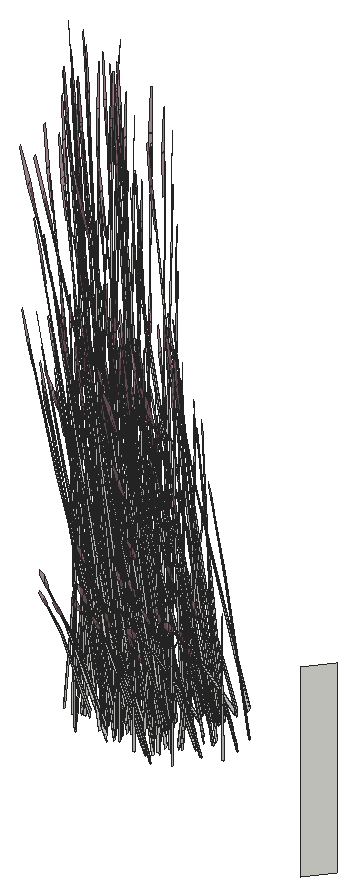
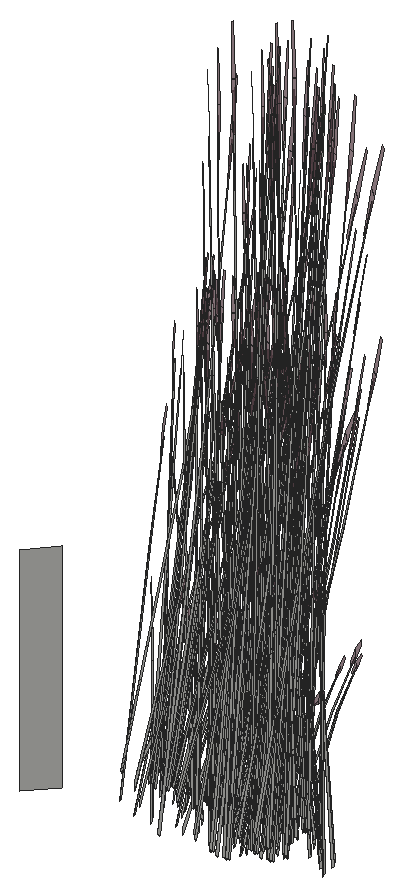
# SketchUp Ruby script. Lengths in inches.
U = 1.inch
M = Sketchup.active_model
def pt(a) = Geom::Point3d.new(a.map { |v| v * U })
def face(e, loops, mat)
  f = e.add_face(loops[0].map { |a| pt(a) })
  loops[1..].each { |l| e.add_face(l.map { |a| pt(a) }).erase! }
  f.material = f.back_material = mat if mat
  f
end
# faces: each face lists its corners as indices into pts; further lists are holes
def faces(e, pts, list, mat = nil) = list.each { |f| face(e, (f[0].is_a?(Array) ? f : [f]).map { |l| l.map { |i| pts[i] } }, mat) }
# xy, xz, yz: faces in a plane at the given z, y or x. An outline is a flat list of corners, or four numbers for a rectangle; further outlines are holes
def ring(l) = l.size == 4 ? [[l[0], l[1]], [l[2], l[1]], [l[2], l[3]], [l[0], l[3]]] : l.each_slice(2).to_a
def flat(e, list, mat, &to3) = list.each { |f| face(e, (f[0].is_a?(Array) ? f : [f]).map { |l| ring(l).map { |u, v| to3.(u, v) } }, mat) }
def xy(e, z, list, mat = nil) = flat(e, list, mat) { |x, y| [x, y, z] }
def xz(e, y, list, mat = nil) = flat(e, list, mat) { |x, z| [x, y, z] }
def yz(e, x, list, mat = nil) = flat(e, list, mat) { |y, z| [x, y, z] }
def lines(e, pts, list) = list.each { |a, b| e.add_line(pt(pts[a]), pt(pts[b])) }
# prism: a flat outline (further loops are holes) pulled along v
def prism(e, loops, v, mat = nil)
  f = face(e, loops, mat); d = Geom::Vector3d.new(v.map { |x| x * U })
  f.pushpull(f.normal.samedirection?(d) ? d.length : -d.length)
end
def box(e, o, s, mat = nil) = prism(e, [[o, [o[0] + s[0], o[1], o[2]], [o[0] + s[0], o[1] + s[1], o[2]], [o[0], o[1] + s[1], o[2]]]], [0, 0, s[2]], mat)
def at(x, y, z, deg = 0) = Geom::Transformation.translation(pt([x, y, z])) * Geom::Transformation.rotation(ORIGIN, Z_AXIS, deg.degrees)
def axes(o, x, y, z) = Geom::Transformation.new([*x, 0, *y, 0, *z, 0, *pt(o).to_a, 1])
def part(name) = M.definitions.add(name)
# library, detail: a bought-in or finely detailed component or shape, given as its bounding box
def library(name, o, s) = part(name).tap { |d| box(d.entities, o, s) }
def detail(e, o, s) = box(e.add_group.entities, o, s)
def put(e, d, t, mat = nil) = e.add_instance(d, t).tap { |i| i.material = mat if mat }
def group(e, t, mat = nil) = e.add_group.tap { |g| g.transformation = t; g.material = mat if mat }.entities
root = M.entities
M.materials.add("LightPink_Translucent").color = [144, 107, 117]
M.materials["LightPink_Translucent"].alpha = 0.75
c1 = part("blade")
p = [[2.15,0.21,22],[0,0.17,0],[0.09,0.45,0],[2.18,0.31,22],[2.29,0.31,22],[0.38,0.45,0],
  [2.48,0.24,33],[2.49,0.24,33],[2.48,0.22,33]]
faces(c1.entities,p,[[0,1,2,3],[4,5,2,3],[6,3,4,7],[8,0,3,6]])
c2 = part("seeds")
p = [[0.3,-0.1,1.38],[-0.01,-0.03,1.59],[-0.01,-0.03,0.03],[0.14,-0.07,-0.07],[0.29,-0.03,3],[0.15,0.01,3.11]]
faces(c2.entities,p,[[0,1,2,3],[1,0,4,5]],"LightPink_Translucent")
c3 = part("blade with seeds")
put(c3.entities,c1,at(0,0,0))
put(c3.entities,c2,axes([2.4,0.25,30.99],[1.5799,-0.05474,1.17369],[-0.12525,1.92788,0.29478],[-0.07173,-0.02425,1.56792]))
p = [[371.24,649.12,618],[369.42,647.05,618],[369.42,647.05,636],[371.24,649.12,636]]
faces(root,p,[[0,1,2,3]])
put(root,c3,axes([347.8,648.96,622.99],[0.18411,0.16231,1.1486],[-0.26813,0.09757,0.84392],[-0.05737,-0.12474,0.25299]))
put(root,c3,axes([349.17,649.44,624.96],[0.26007,-0.1585,0.0643],[0.12729,0.28902,0.50621],[-0.02512,-0.1274,0.77189]))
put(root,c3,axes([349.38,649.62,624.78],[0.39316,-0.11987,0.53763],[0.06823,0.47021,0.4433],[-0.09247,-0.13858,1.11249]))
put(root,c3,axes([352.93,649.92,620.63],[-0.0592,0.0168,1.76342],[-0.32738,-0.18913,-0.26939],[0.00549,-0.15776,0.30037]))
put(root,c3,axes([350.27,649.71,624.42],[0.34777,0.12192,0.48003],[-0.11892,0.40083,0.3958],[-0.0209,-0.15763,0.9933]))
put(root,c3,axes([350.37,649.85,624.73],[-0.34538,0.21713,-0.1216],[-0.16972,-0.38536,-0.67495],[-0.04557,-0.16239,1.02557]))
put(root,c3,axes([351.09,650.34,624.73],[-0.3879,-0.02311,-0.1216],[0.0106,-0.43749,-0.67495],[0.02694,-0.1685,1.02557]))
put(root,c3,axes([351.0625,650.06,624.22],[0.23881,-0.24554,-0.35414],[0.22606,0.28036,0.4572],[0.0344,-0.14245,0.87481]))
put(root,c3,axes([349,649.19,622.46],[0.18411,0.16231,1.1486],[-0.26813,0.09757,0.84392],[-0.05737,-0.12474,0.25299]))
put(root,c3,axes([350.36,649.68,624.42],[0.26007,-0.1585,0.0643],[0.12729,0.28902,0.50621],[-0.02512,-0.1274,0.77189]))
put(root,c3,axes([353.92,651.13,624.12],[0.00918,-0.43138,-0.71045],[0.38672,0.02897,0.08574],[0.04081,-0.18275,1.00501]))
put(root,c3,axes([349.44,650.05,624.67],[-0.30095,-0.22541,-0.71045],[0.21388,-0.395,0.08574],[-0.10904,-0.13459,1.00501]))
put(root,c3,axes([349.34,649.76,624.22],[-0.05451,-0.37564,-0.35414],[0.31161,-0.09919,0.4572],[-0.0837,-0.10765,0.87481]))
put(root,c3,axes([354.46,650.46,623.85],[-0.00341,-0.09282,1.74944],[-0.28775,-0.26825,-0.27667],[0.04449,-0.16261,0.14031]))
put(root,c3,axes([353.25,650.4375,623.66],[0.1064,-0.35863,-0.35414],[0.31043,0.1046,0.4572],[-0.02846,-0.14439,0.87481]))
put(root,c3,axes([353.48,650.91,623.01],[-0.06572,0.16029,1.71376],[-0.27569,-0.33172,0.13857],[0.12437,-0.20675,0.73262]))
put(root,c3,axes([354.38,650.125,623.85],[-0.03584,0.03562,1.77383],[-0.35118,-0.12018,-0.16761],[-0.01271,-0.15545,0.31391]))
put(root,c3,axes([346.05,649.49,621.22],[-0.05283,-0.03674,1.76342],[-0.13569,-0.41045,-0.26939],[0.09154,-0.11138,0.30037]))
put(root,c3,axes([348.28,649.48,624.96],[0.16041,-0.29625,0.0643],[0.22843,0.17248,0.50621],[-0.07385,-0.09498,0.77189]))
put(root,c3,axes([348.23,651.13,622.32],[-0.14494,-0.47823,-0.69835],[0.41752,-0.17223,-0.18329],[-0.01602,-0.16194,1.54149]))
put(root,c3,axes([353.09,650.68,623.82],[-0.34695,-0.11691,-0.51099],[0.11892,-0.40083,-0.3958],[-0.03181,-0.16138,0.97773]))
put(root,c3,axes([350.17,649.67,621.72],[-0.05283,-0.03674,1.76342],[-0.13569,-0.41045,-0.26939],[0.09154,-0.11138,0.30037]))
put(root,c3,axes([353.31,649.68,621.9],[0.04528,0.27194,1.1486],[-0.25117,-0.15062,0.84392],[0.02703,-0.13924,0.25299]))
put(root,c3,axes([345.75,649.74,624.46],[0.25132,0.3182,0.48003],[-0.2669,0.27442,0.3958],[0.04636,-0.14929,0.9933]))
put(root,c3,axes([353.84,650.99,623.82],[-0.25266,-0.31335,-0.51099],[0.2669,-0.27442,-0.3958],[0.03844,-0.15921,0.97773]))
put(root,c3,axes([349.47,649.72,624.42],[0.16041,-0.29625,0.0643],[0.22843,0.17248,0.50621],[-0.07385,-0.09498,0.77189]))
put(root,c3,axes([348.85,649.68,621.18],[-0.03419,0.06144,1.76342],[-0.3455,0.13246,-0.26939],[-0.08346,-0.12049,0.30037]))
put(root,c3,axes([349.07,649.77,625.28],[-0.1064,0.35863,0.35414],[-0.31043,-0.1046,-0.4572],[-0.02846,-0.14439,0.87481]))
put(root,c3,axes([352.47,649.44,623.85],[-0.00658,0.0559,1.77383],[-0.32474,0.20287,-0.16761],[-0.09556,-0.1037,0.31391]))
put(root,c3,axes([349.42,651.37,621.79],[-0.14494,-0.47823,-0.69835],[0.41752,-0.17223,-0.18329],[-0.01602,-0.16194,1.54149]))
put(root,c3,axes([349.87,649.92,624.96],[0.25132,0.3182,0.48003],[-0.2669,0.27442,0.3958],[0.04636,-0.14929,0.9933]))
put(root,c3,axes([351.36,649.91,621.18],[-0.05283,-0.03674,1.76342],[-0.13569,-0.41045,-0.26939],[0.09154,-0.11138,0.30037]))
put(root,c3,axes([346.05,650.65,624.71],[0.18436,-0.36797,-0.71045],[0.32306,0.26151,0.08574],[0.11008,-0.13332,1.00501]))
put(root,c3,axes([349.96,649.95,624.96],[0.29004,0.02173,0.0643],[-0.00795,0.32812,0.50621],[0.03035,-0.12569,0.77189]))
put(root,c3,axes([346.04,650.48,624.41],[-0.09067,-0.42583,-0.51099],[0.34336,-0.07449,-0.3958],[0.0984,-0.11438,0.97773]))
put(root,c3,axes([352.4,650.43,624.23],[0.39316,-0.11987,0.53763],[0.06823,0.47021,0.4433],[-0.09247,-0.13858,1.11249]))
put(root,c3,axes([350.27,650,624.74],[-0.1064,0.35863,0.35414],[-0.31043,-0.1046,-0.4572],[-0.02846,-0.14439,0.87481]))
put(root,c3,axes([349.74,650.17,625.28],[-0.23881,0.24554,0.35414],[-0.22606,-0.28036,-0.4572],[0.0344,-0.14245,0.87481]))
put(root,c3,axes([353.29,650.52,623.87],[0.34777,0.12192,0.48003],[-0.11892,0.40083,0.3958],[-0.0209,-0.15763,0.9933]))
put(root,c3,axes([350.16,650.83,625.21],[0.18436,-0.36797,-0.71045],[0.32306,0.26151,0.08574],[0.11008,-0.13332,1.00501]))
put(root,c3,axes([348.17,649.76,622.6],[-0.22066,-0.46731,0],[0.36918,-0.26061,-0.51607],[0.08408,-0.05936,1.63711]))
put(root,c3,axes([350.16,650.66,624.91],[-0.09067,-0.42583,-0.51099],[0.34336,-0.07449,-0.3958],[0.0984,-0.11438,0.97773]))
put(root,c3,axes([353.39,650.66,624.17],[-0.34538,0.21713,-0.1216],[-0.16972,-0.38536,-0.67495],[-0.04557,-0.16239,1.02557]))
put(root,c3,axes([349.3,650.07,624.37],[-0.34827,0.11086,-0.51099],[-0.06092,-0.41983,-0.3958],[-0.09354,-0.12031,0.97773]))
put(root,c3,axes([351.0625,650.15,624.42],[0.25132,0.3182,0.48003],[-0.2669,0.27442,0.3958],[0.04636,-0.14929,0.9933]))
put(root,c3,axes([354.11,651.15,624.17],[-0.3879,-0.02311,-0.1216],[0.0106,-0.43749,-0.67495],[0.02694,-0.1685,1.02557]))
put(root,c3,axes([346.2,650.78,624.76],[-0.32648,-0.25715,-0.1216],[0.18809,-0.3724,-0.67495],[0.09224,-0.12945,1.02557]))
put(root,c3,axes([349.55,649.69,625.12],[-0.23555,0.44708,-0.13619],[-0.34112,-0.25757,-0.75594],[-0.11858,-0.12631,1.14864]))
put(root,c3,axes([354.08,650.87,623.66],[0.23881,-0.24554,-0.35414],[0.22606,0.28036,0.4572],[0.0344,-0.14245,0.87481]))
put(root,c3,axes([352.01,650.01,621.9],[0.18411,0.16231,1.1486],[-0.26813,0.09757,0.84392],[-0.05737,-0.12474,0.25299]))
put(root,c3,axes([351.15,650.18,624.42],[0.29004,0.02173,0.0643],[-0.00795,0.32812,0.50621],[0.03035,-0.12569,0.77189]))
put(root,c3,axes([353.38,650.49,623.87],[0.26007,-0.1585,0.0643],[0.12729,0.28902,0.50621],[-0.02512,-0.1274,0.77189]))
put(root,c3,axes([348.66,649.2,622.35],[-0.2439,0.26754,-0.03893],[-0.22348,-0.29302,-0.17649],[-0.01573,-0.08303,0.58215]))
put(root,c3,axes([352.46,650.87,624.12],[-0.30095,-0.22541,-0.71045],[0.21388,-0.395,0.08574],[-0.10904,-0.13459,1.00501]))
put(root,c3,axes([352.35,650.57,623.66],[-0.05451,-0.37564,-0.35414],[0.31161,-0.09919,0.4572],[-0.0837,-0.10765,0.87481]))
put(root,c3,axes([350.9375,650.41,624.74],[-0.23881,0.24554,0.35414],[-0.22606,-0.28036,-0.4572],[0.0344,-0.14245,0.87481]))
put(root,c3,axes([350.32,650.96,625.26],[-0.32648,-0.25715,-0.1216],[0.18809,-0.3724,-0.67495],[0.09224,-0.12945,1.02557]))
put(root,c3,axes([351.36,651.07,624.67],[0.18436,-0.36797,-0.71045],[0.32306,0.26151,0.08574],[0.11008,-0.13332,1.00501]))
put(root,c3,axes([349.37,650,622.0625],[-0.22066,-0.46731,0],[0.36918,-0.26061,-0.51607],[0.08408,-0.05936,1.63711]))
put(root,c3,axes([351.35,650.9,624.37],[-0.09067,-0.42583,-0.51099],[0.34336,-0.07449,-0.3958],[0.0984,-0.11438,0.97773]))
put(root,c3,axes([355.77,652.23,624.04],[0.08068,0.14973,1.71376],[-0.3728,0.12606,0.13857],[-0.08426,-0.23506,0.73262]))
put(root,c3,axes([349.85,649.43,621.82],[-0.2439,0.26754,-0.03893],[-0.22348,-0.29302,-0.17649],[-0.01573,-0.08303,0.58215]))
put(root,c3,axes([344.38,650.3125,622.3],[-0.12609,-0.01381,1.43002],[-0.12917,-0.37055,-0.30754],[0.1549,-0.10482,0.61141]))
put(root,c3,axes([346.32,650.3125,622.32],[-0.12609,-0.01381,1.43002],[-0.12917,-0.37055,-0.30754],[0.1549,-0.10482,0.61141]))
put(root,c3,axes([356.39,651.24,624.88],[-0.05398,-0.06539,1.74944],[-0.36026,0.04145,-0.27667],[-0.0575,-0.15639,0.14031]))
put(root,c3,axes([347.01,650.67,624.43],[-0.0461,-0.00354,1.77383],[-0.19143,-0.37951,-0.16761],[0.07688,-0.12478,0.31391]))
put(root,c3,axes([348.97,652.37,623.55],[0.305,0.18805,1.51261],[-0.29879,0.40513,0.59816],[-0.13384,-0.24012,1.26806]))
put(root,c3,axes([357.22,652.01,622.76],[-0.10032,0.0944,1.43002],[-0.30046,-0.16522,-0.30754],[0.05569,-0.20547,0.61141]))
put(root,c3,axes([351.51,651.2,624.73],[-0.32648,-0.25715,-0.1216],[0.18809,-0.3724,-0.67495],[0.09224,-0.12945,1.02557]))
put(root,c3,axes([352.49,650.53,623.87],[0.16041,-0.29625,0.0643],[0.22843,0.17248,0.50621],[-0.07385,-0.09498,0.77189]))
put(root,c3,axes([351.87,650.5,620.63],[-0.03419,0.06144,1.76342],[-0.3455,0.13246,-0.26939],[-0.08346,-0.12049,0.30037]))
put(root,c3,axes([356.77,652.34,625.15],[-0.16845,-0.3792,-0.71045],[0.34676,-0.21133,0.08574],[-0.03939,-0.18322,1.00501]))
put(root,c3,axes([348.33,649.83,625.28],[0.05451,0.37564,0.35414],[-0.31161,0.09919,-0.4572],[-0.0837,-0.10765,0.87481]))
put(root,c3,axes([344.75,650.46,621.78],[0.23773,-0.35053,-0.62353],[0.29532,0.31785,-0.16365],[0.09526,-0.08744,1.37633]))
put(root,c3,axes([346.46,649.63,622.49],[-0.11756,0.2374,1.1486],[-0.10105,-0.31895,0.84392],[0.09709,-0.07992,0.25299]))
put(root,c3,axes([347.375,651.07,622.24],[0,-0.46636,-0.49651],[0.39487,0,0],[0,-0.10622,1.57504]))
put(root,c3,axes([348.47,649.6875,622.24],[0.33032,-0.23318,-0.49651],[0.19744,0.41812,0],[0.07523,-0.05311,1.57504]))
put(root,c3,axes([350.43,650.49,622.82],[-0.12609,-0.01381,1.43002],[-0.12917,-0.37055,-0.30754],[0.1549,-0.10482,0.61141]))
put(root,c3,axes([351.12,650.85,624.93],[-0.0461,-0.00354,1.77383],[-0.19143,-0.37951,-0.16761],[0.07688,-0.12478,0.31391]))
put(root,c3,axes([355.67,651.84,622.76],[-0.02137,0.15256,1.43002],[-0.31245,0.12771,-0.30754],[-0.07303,-0.19719,0.61141]))
put(root,c3,axes([352.4375,652.18,621.24],[-0.14494,-0.47823,-0.69835],[0.41752,-0.17223,-0.18329],[-0.01602,-0.16194,1.54149]))
put(root,c3,axes([351.68,651.12,623.01],[0.1311,0.08035,1.71376],[-0.27131,0.33708,0.13857],[-0.16909,-0.15206,0.73262]))
put(root,c3,axes([354.375,650.72,620.63],[-0.05283,-0.03674,1.76342],[-0.13569,-0.41045,-0.26939],[0.09154,-0.11138,0.30037]))
put(root,c3,axes([350.16,652.6,623.02],[0.305,0.18805,1.51261],[-0.29879,0.40513,0.59816],[-0.13384,-0.24012,1.26806]))
put(root,c3,axes([348.86,650.64,622.28],[0.23773,-0.35053,-0.62353],[0.29532,0.31785,-0.16365],[0.09526,-0.08744,1.37633]))
put(root,c3,axes([356.48,651.5,621.66],[-0.0592,0.0168,1.76342],[-0.32738,-0.18913,-0.26939],[0.00549,-0.15776,0.30037]))
put(root,c3,axes([350.58,649.8125,622.99],[-0.11756,0.2374,1.1486],[-0.10105,-0.31895,0.84392],[0.09709,-0.07992,0.25299]))
put(root,c3,axes([346.29,650.52,624.25],[0.30722,-0.06665,-0.35414],[0.08112,0.381,0.4572],[0.08804,-0.10234,0.87481]))
put(root,c3,axes([349.52,650.0625,624.74],[0.05451,0.37564,0.35414],[-0.31161,0.09919,-0.4572],[-0.0837,-0.10765,0.87481]))
put(root,c3,axes([353.28,650.82,624.1875],[-0.1064,0.35863,0.35414],[-0.31043,-0.1046,-0.4572],[-0.02846,-0.14439,0.87481]))
put(root,c3,axes([348.57,651.3,621.71],[0,-0.46636,-0.49651],[0.39487,0,0],[0,-0.10622,1.57504]))
put(root,c3,axes([349.67,649.92,621.71],[0.33032,-0.23318,-0.49651],[0.19744,0.41812,0],[0.07523,-0.05311,1.57504]))
put(root,c3,axes([351.625,650.73,622.28],[-0.12609,-0.01381,1.43002],[-0.12917,-0.37055,-0.30754],[0.1549,-0.10482,0.61141]))
put(root,c3,axes([352.32,651.09,624.4],[-0.0461,-0.00354,1.77383],[-0.19143,-0.37951,-0.16761],[0.07688,-0.12478,0.31391]))
put(root,c3,axes([352.32,650.88,623.82],[-0.34827,0.11086,-0.51099],[-0.06092,-0.41983,-0.3958],[-0.09354,-0.12031,0.97773]))
put(root,c3,axes([354.08,650.97,623.87],[0.25132,0.3182,0.48003],[-0.2669,0.27442,0.3958],[0.04636,-0.14929,0.9933]))
put(root,c3,axes([357.47,652.71,625.15],[0.00918,-0.43138,-0.71045],[0.38672,0.02897,0.08574],[0.04081,-0.18275,1.00501]))
put(root,c3,axes([352.5625,650.5,624.57],[-0.23555,0.44708,-0.13619],[-0.34112,-0.25757,-0.75594],[-0.11858,-0.12631,1.14864]))
put(root,c3,axes([354.17,651,623.87],[0.29004,0.02173,0.0643],[-0.00795,0.32812,0.50621],[0.03035,-0.12569,0.77189]))
put(root,c3,axes([350.41,650.7,624.75],[0.30722,-0.06665,-0.35414],[0.08112,0.381,0.4572],[0.08804,-0.10234,0.87481]))
put(root,c3,axes([350.06,650.88,621.75],[0.23773,-0.35053,-0.62353],[0.29532,0.31785,-0.16365],[0.09526,-0.08744,1.37633]))
put(root,c3,axes([351.77,650.05,622.46],[-0.11756,0.2374,1.1486],[-0.10105,-0.31895,0.84392],[0.09709,-0.07992,0.25299]))
put(root,c3,axes([358.01,652.04,624.88],[-0.00341,-0.09282,1.74944],[-0.28775,-0.26825,-0.27667],[0.04449,-0.16261,0.14031]))
put(root,c3,axes([356.8,652.02,624.7],[0.1064,-0.35863,-0.35414],[0.31043,0.1046,0.4572],[-0.02846,-0.14439,0.87481]))
put(root,c3,axes([346.04,650.75,624.78],[-0.30722,0.06665,0.35414],[-0.08112,-0.381,-0.4572],[0.08804,-0.10234,0.87481]))
put(root,c3,axes([357.03,652.5,624.04],[-0.06572,0.16029,1.71376],[-0.27569,-0.33172,0.13857],[0.12437,-0.20675,0.73262]))
put(root,c3,axes([357.93,651.71,624.88],[-0.03584,0.03562,1.77383],[-0.35118,-0.12018,-0.16761],[-0.01271,-0.15545,0.31391]))
put(root,c3,axes([353.95,651.22,624.1875],[-0.23881,0.24554,0.35414],[-0.22606,-0.28036,-0.4572],[0.0344,-0.14245,0.87481]))
put(root,c3,axes([348.45,651.26,622.4375],[0.17124,-0.42022,-0.44739],[0.35581,0.20224,0.21531],[0,-0.09687,1.43643]))
put(root,c3,axes([354.375,651.88,624.12],[0.18436,-0.36797,-0.71045],[0.32306,0.26151,0.08574],[0.11008,-0.13332,1.00501]))
put(root,c3,axes([348.61,651.05,622.89],[-0.04113,-0.53214,-0.29095],[0.42835,-0.03218,-0.50002],[0.07543,-0.07088,1.59708]))
put(root,c3,axes([352.38,650.81,621.51],[-0.22066,-0.46731,0],[0.36918,-0.26061,-0.51607],[0.08408,-0.05936,1.63711]))
put(root,c3,axes([354.37,651.71,623.82],[-0.09067,-0.42583,-0.51099],[0.34336,-0.07449,-0.3958],[0.0984,-0.11438,0.97773]))
put(root,c3,axes([347.54,651.08,622.25],[0.24637,-0.29097,-0.30978],[0.24637,0.29097,0.30978],[0,-0.09372,1.38974]))
put(root,c3,axes([352.87,650.25,621.27],[-0.2439,0.26754,-0.03893],[-0.22348,-0.29302,-0.17649],[-0.01573,-0.08303,0.58215]))
put(root,c3,axes([351.6,650.94,624.22],[0.30722,-0.06665,-0.35414],[0.08112,0.381,0.4572],[0.08804,-0.10234,0.87481]))
put(root,c3,axes([350.16,650.93,625.28],[-0.30722,0.06665,0.35414],[-0.08112,-0.381,-0.4572],[0.08804,-0.10234,0.87481]))
put(root,c3,axes([356.64,652.27,624.85],[-0.34695,-0.11691,-0.51099],[0.11892,-0.40083,-0.3958],[-0.03181,-0.16138,0.97773]))
put(root,c3,axes([348.41,651.61,622.89],[-0.39748,-0.22252,-0.29095],[0.19139,-0.46966,-0.50002],[-0.01249,-0.11531,1.59708]))
put(root,c3,axes([356.85,651.26,622.93],[0.04528,0.27194,1.1486],[-0.25117,-0.15062,0.84392],[0.02703,-0.13924,0.25299]))
put(root,c3,axes([348.72,650.3,624.42],[0.01777,-0.35463,0.0643],[0.26836,0.00972,0.50621],[-0.1028,-0.03711,0.77189]))
put(root,c3,axes([349.64,651.49,621.9],[0.17124,-0.42022,-0.44739],[0.35581,0.20224,0.21531],[0,-0.09687,1.43643]))
put(root,c3,axes([357.39,652.57,624.85],[-0.25266,-0.31335,-0.51099],[0.2669,-0.27442,-0.3958],[0.03844,-0.15921,0.97773]))
put(root,c3,axes([351.66,650.375,623.85],[-0.07594,-0.00329,1.74944],[-0.24177,0.32918,-0.27667],[-0.129,-0.06726,0.14031]))
put(root,c3,axes([354.53,652.01,624.17],[-0.32648,-0.25715,-0.1216],[0.18809,-0.3724,-0.67495],[0.09224,-0.12945,1.02557]))
put(root,c3,axes([349.8,651.29,622.36],[-0.04113,-0.53214,-0.29095],[0.42835,-0.03218,-0.50002],[0.07543,-0.07088,1.59708]))
put(root,c3,axes([348.74,651.31,621.72],[0.24637,-0.29097,-0.30978],[0.24637,0.29097,0.30978],[0,-0.09372,1.38974]))
put(root,c3,axes([356.02,651.02,624.88],[-0.00658,0.0559,1.77383],[-0.32474,0.20287,-0.16761],[-0.09556,-0.1037,0.31391]))
put(root,c3,axes([348.55,649.87,622.25],[0.32928,0.11539,-0.30978],[-0.08291,0.40636,0.30978],[0.06638,-0.04686,1.38974]))
put(root,c3,axes([348.64,649.92,621.82],[-0.10181,0.3808,-0.03893],[-0.31336,-0.11714,-0.17649],[-0.04758,-0.06228,0.58215]))
put(root,c3,axes([351.35,651.17,624.74],[-0.30722,0.06665,0.35414],[-0.08112,-0.381,-0.4572],[0.08804,-0.10234,0.87481]))
put(root,c3,axes([349.6,651.84,622.36],[-0.39748,-0.22252,-0.29095],[0.19139,-0.46966,-0.50002],[-0.01249,-0.11531,1.59708]))
put(root,c3,axes([346.32,650.6875,624.46],[0.2423,0.19613,0.0643],[-0.14107,0.2793,0.50621],[0.07768,-0.0903,0.77189]))
put(root,c3,axes([348.47,651.66,622.0625],[-0.44133,0,0],[0,-0.52122,-0.51607],[0,-0.11871,1.63711]))
put(root,c3,axes([346.25,650.61,624.46],[0.08753,0.42921,0.48003],[-0.34336,0.07449,0.3958],[0.1012,-0.10094,0.9933]))
put(root,c3,axes([353.18,653.42,622.46],[0.305,0.18805,1.51261],[-0.29879,0.40513,0.59816],[-0.13384,-0.24012,1.26806]))
put(root,c3,axes([355.95,652.02,625.26],[0.39316,-0.11987,0.53763],[0.06823,0.47021,0.4433],[-0.09247,-0.13858,1.11249]))
put(root,c3,axes([345.25,651.125,624.42],[0.04898,-0.07104,1.74944],[-0.06269,-0.43574,-0.27667],[0.12289,-0.08262,0.14031]))
put(root,c3,axes([347.18,651.125,624.44],[0.04898,-0.07104,1.74944],[-0.06269,-0.43574,-0.27667],[0.12289,-0.08262,0.14031]))
put(root,c3,axes([352.54,650.875,624.1875],[0.05451,0.37564,0.35414],[-0.31161,0.09919,-0.4572],[-0.0837,-0.10765,0.87481]))
put(root,c3,axes([356.84,652.1,624.9],[0.34777,0.12192,0.48003],[-0.11892,0.40083,0.3958],[-0.0209,-0.15763,0.9933]))
put(root,c3,axes([349.74,650.11,621.72],[0.32928,0.11539,-0.30978],[-0.08291,0.40636,0.30978],[0.06638,-0.04686,1.38974]))
put(root,c3,axes([351.58,652.12,621.16],[0,-0.46636,-0.49651],[0.39487,0,0],[0,-0.10622,1.57504]))
put(root,c3,axes([352.68,650.74,621.16],[0.33032,-0.23318,-0.49651],[0.19744,0.41812,0],[0.07523,-0.05311,1.57504]))
put(root,c3,axes([356.9375,652.25,625.2],[-0.34538,0.21713,-0.1216],[-0.16972,-0.38536,-0.67495],[-0.04557,-0.16239,1.02557]))
put(root,c3,axes([354.64,651.54,621.73],[-0.12609,-0.01381,1.43002],[-0.12917,-0.37055,-0.30754],[0.1549,-0.10482,0.61141]))
put(root,c3,axes([351.6,651.12,624.23],[0.29147,-0.34417,0.53763],[0.25138,0.3655,0.4433],[-0.13675,-0.06349,1.11249]))
put(root,c3,axes([355.33,651.9,623.85],[-0.0461,-0.00354,1.77383],[-0.19143,-0.37951,-0.16761],[0.07688,-0.12478,0.31391]))
put(root,c3,axes([357.65,652.74,625.2],[-0.3879,-0.02311,-0.1216],[0.0106,-0.43749,-0.67495],[0.02694,-0.1685,1.02557]))
put(root,c3,axes([350.4375,650.87,624.96],[0.2423,0.19613,0.0643],[-0.14107,0.2793,0.50621],[0.07768,-0.0903,0.77189]))
put(root,c3,axes([357.63,652.45,624.7],[0.23881,-0.24554,-0.35414],[0.22606,0.28036,0.4572],[0.0344,-0.14245,0.87481]))
put(root,c3,axes([355.5625,651.59,622.93],[0.18411,0.16231,1.1486],[-0.26813,0.09757,0.84392],[-0.05737,-0.12474,0.25299]))
put(root,c3,axes([350.37,650.79,624.96],[0.08753,0.42921,0.48003],[-0.34336,0.07449,0.3958],[0.1012,-0.10094,0.9933]))
put(root,c3,axes([356.93,652.07,624.9],[0.26007,-0.1585,0.0643],[0.12729,0.28902,0.50621],[-0.02512,-0.1274,0.77189]))
put(root,c3,axes([356.01,652.45,625.15],[-0.30095,-0.22541,-0.71045],[0.21388,-0.395,0.08574],[-0.10904,-0.13459,1.00501]))
put(root,c3,axes([351.3,651.3,624.94],[0.04898,-0.07104,1.74944],[-0.06269,-0.43574,-0.27667],[0.12289,-0.08262,0.14031]))
put(root,c3,axes([355.9,652.15,624.7],[-0.05451,-0.37564,-0.35414],[0.31161,-0.09919,0.4572],[-0.0837,-0.10765,0.87481]))
put(root,c3,axes([353.07,651.69,621.2],[0.23773,-0.35053,-0.62353],[0.29532,0.31785,-0.16365],[0.09526,-0.08744,1.37633]))
put(root,c3,axes([354.79,650.86,621.9],[-0.11756,0.2374,1.1486],[-0.10105,-0.31895,0.84392],[0.09709,-0.07992,0.25299]))
put(root,c3,axes([358.06,653.76,624.72],[0.08068,0.14973,1.71376],[-0.3728,0.12606,0.13857],[-0.08426,-0.23506,0.73262]))
put(root,c3,axes([347.62,651.28,622.56],[-0.32829,0.39208,0.30756],[-0.32849,-0.38796,-0.36492],[-0.01146,-0.11134,1.64885]))
put(root,c3,axes([351.63,651.11,624.42],[0.2423,0.19613,0.0643],[-0.14107,0.2793,0.50621],[0.07768,-0.0903,0.77189]))
put(root,c3,axes([351.5625,651.02,624.42],[0.08753,0.42921,0.48003],[-0.34336,0.07449,0.3958],[0.1012,-0.10094,0.9933]))
put(root,c3,axes([358.67,652.77,625.56],[-0.05398,-0.06539,1.74944],[-0.36026,0.04145,-0.27667],[-0.0575,-0.15639,0.14031]))
put(root,c3,axes([352.49,651.54,624.41],[0.04898,-0.07104,1.74944],[-0.06269,-0.43574,-0.27667],[0.12289,-0.08262,0.14031]))
put(root,c3,axes([354.62,651.75,623.66],[0.30722,-0.06665,-0.35414],[0.08112,0.381,0.4572],[0.08804,-0.10234,0.87481]))
put(root,c3,axes([359.51,653.54,623.4375],[-0.10032,0.0944,1.43002],[-0.30046,-0.16522,-0.30754],[0.05569,-0.20547,0.61141]))
put(root,c3,axes([348.66,651.47,622.66],[0.39767,0.22603,0.24065],[-0.19139,0.46966,0.50002],[0,-0.10827,1.60543]))
put(root,c3,axes([351.74,651.12,623.87],[0.01777,-0.35463,0.0643],[0.26836,0.00972,0.50621],[-0.1028,-0.03711,0.77189]))
put(root,c3,axes([348.51,652.1,622.66],[0.09355,-0.55261,-0.23429],[0.44354,0.09633,0.51271],[-0.0775,-0.07631,1.5644]))
put(root,c3,axes([359.05,653.87,625.83],[-0.16845,-0.3792,-0.71045],[0.34676,-0.21133,0.08574],[-0.03939,-0.18322,1.00501]))
put(root,c3,axes([352.66,652.31,621.35],[0.17124,-0.42022,-0.44739],[0.35581,0.20224,0.21531],[0,-0.09687,1.43643]))
put(root,c3,axes([351.63,651.23,623.66],[-0.20082,-0.29199,-0.35414],[0.2293,-0.2764,0.4572],[-0.1165,-0.04206,0.87481]))
put(root,c3,axes([348.8125,651.52,622.02],[-0.32829,0.39208,0.30756],[-0.32849,-0.38796,-0.36492],[-0.01146,-0.11134,1.64885]))
put(root,c3,axes([356.04,652.12,624.9],[0.16041,-0.29625,0.0643],[0.22843,0.17248,0.50621],[-0.07385,-0.09498,0.77189]))
put(root,c3,axes([355.42,652.08,621.66],[-0.03419,0.06144,1.76342],[-0.3455,0.13246,-0.26939],[-0.08346,-0.12049,0.30037]))
put(root,c3,axes([357.96,653.36,623.4375],[-0.02137,0.15256,1.43002],[-0.31245,0.12771,-0.30754],[-0.07303,-0.19719,0.61141]))
put(root,c3,axes([352.82,652.1,621.8],[-0.04113,-0.53214,-0.29095],[0.42835,-0.03218,-0.50002],[0.07543,-0.07088,1.59708]))
put(root,c3,axes([351.75,652.13,621.17],[0.24637,-0.29097,-0.30978],[0.24637,0.29097,0.30978],[0,-0.09372,1.38974]))
put(root,c3,axes([355.99,653.77,622.27],[-0.14494,-0.47823,-0.69835],[0.41752,-0.17223,-0.18329],[-0.01602,-0.16194,1.54149]))
put(root,c3,axes([346.22,651.79,624.76],[-0.17758,-0.42229,-0.1216],[0.31518,-0.20752,-0.67495],[0.13282,-0.05572,1.02557]))
put(root,c3,axes([351.65,650.73,621.27],[-0.10181,0.3808,-0.03893],[-0.31336,-0.11714,-0.17649],[-0.04758,-0.06228,0.58215]))
put(root,c3,axes([355.23,652.7,624.04],[0.1311,0.08035,1.71376],[-0.27131,0.33708,0.13857],[-0.16909,-0.15206,0.73262]))
put(root,c3,axes([344.27,651.42,624.39],[0.09562,-0.42421,-0.51099],[0.32782,0.1454,-0.3958],[0.13199,-0.0389,0.97773]))
put(root,c3,axes([346.2,651.42,624.41],[0.09562,-0.42421,-0.51099],[0.32782,0.1454,-0.3958],[0.13199,-0.0389,0.97773]))
put(root,c3,axes([354.37,651.98,624.1875],[-0.30722,0.06665,0.35414],[-0.08112,-0.381,-0.4572],[0.08804,-0.10234,0.87481]))
put(root,c3,axes([352.62,652.66,621.8],[-0.39748,-0.22252,-0.29095],[0.19139,-0.46966,-0.50002],[-0.01249,-0.11531,1.59708]))
put(root,c3,axes([345.68,649.7,622.1],[0.22066,-0.46731,0],[0.36918,0.26061,-0.51607],[0.08408,0.05936,1.63711]))
put(root,c3,axes([357.93,652.31,621.66],[-0.05283,-0.03674,1.76342],[-0.13569,-0.41045,-0.26939],[0.09154,-0.11138,0.30037]))
put(root,c3,axes([358.76,653.03,622.34],[-0.0592,0.0168,1.76342],[-0.32738,-0.18913,-0.26939],[0.00549,-0.15776,0.30037]))
put(root,c3,axes([349.86,651.7,622.125],[0.39767,0.22603,0.24065],[-0.19139,0.46966,0.50002],[0,-0.10827,1.60543]))
put(root,c3,axes([349.7,652.34,622.13],[0.09355,-0.55261,-0.23429],[0.44354,0.09633,0.51271],[-0.0775,-0.07631,1.5644]))
put(root,c3,axes([351.49,652.47,621.51],[-0.44133,0,0],[0,-0.52122,-0.51607],[0,-0.11871,1.63711]))
put(root,c3,axes([348.53,651.15,622.94],[-0.38326,0.02879,0.44739],[-0.03466,-0.47788,-0.21531],[0.06861,-0.04843,1.43643]))
put(root,c3,axes([347.54,651.5,622.7],[0,0.46636,0.49651],[-0.39487,0,0],[0,-0.10622,1.57504]))
